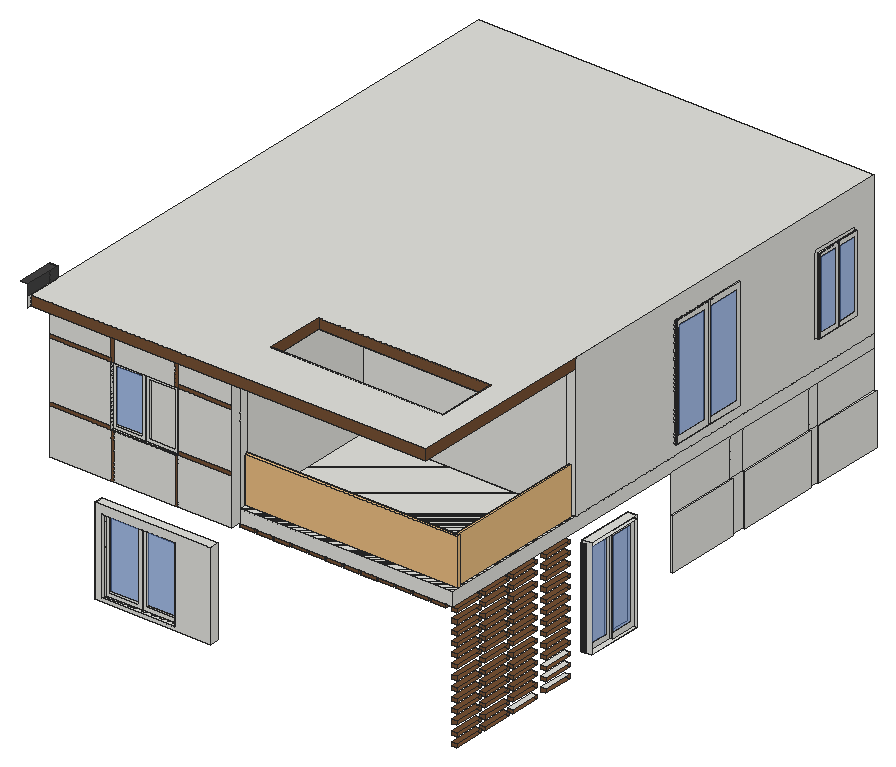
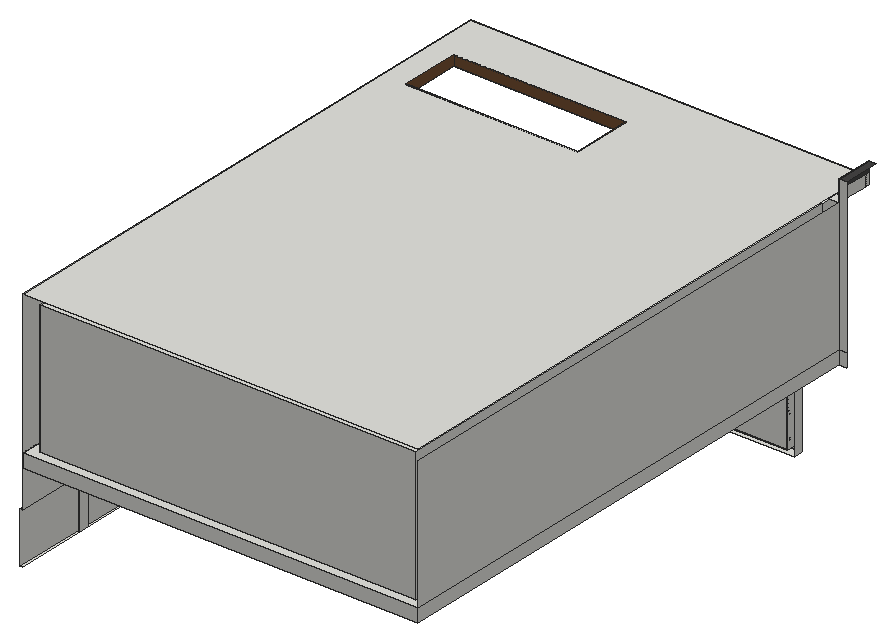
# SketchUp Ruby script. Lengths in inches.
U = 1.inch
M = Sketchup.active_model
def pt(a) = Geom::Point3d.new(a.map { |v| v * U })
def face(e, loops, mat)
  f = e.add_face(loops[0].map { |a| pt(a) })
  loops[1..].each { |l| e.add_face(l.map { |a| pt(a) }).erase! }
  f.material = f.back_material = mat if mat
  f
end
# faces: each face lists its corners as indices into pts; further lists are holes
def faces(e, pts, list, mat = nil) = list.each { |f| face(e, (f[0].is_a?(Array) ? f : [f]).map { |l| l.map { |i| pts[i] } }, mat) }
# xy, xz, yz: faces in a plane at the given z, y or x. An outline is a flat list of corners, or four numbers for a rectangle; further outlines are holes
def ring(l) = l.size == 4 ? [[l[0], l[1]], [l[2], l[1]], [l[2], l[3]], [l[0], l[3]]] : l.each_slice(2).to_a
def flat(e, list, mat, &to3) = list.each { |f| face(e, (f[0].is_a?(Array) ? f : [f]).map { |l| ring(l).map { |u, v| to3.(u, v) } }, mat) }
def xy(e, z, list, mat = nil) = flat(e, list, mat) { |x, y| [x, y, z] }
def xz(e, y, list, mat = nil) = flat(e, list, mat) { |x, z| [x, y, z] }
def yz(e, x, list, mat = nil) = flat(e, list, mat) { |y, z| [x, y, z] }
def lines(e, pts, list) = list.each { |a, b| e.add_line(pt(pts[a]), pt(pts[b])) }
# prism: a flat outline (further loops are holes) pulled along v
def prism(e, loops, v, mat = nil)
  f = face(e, loops, mat); d = Geom::Vector3d.new(v.map { |x| x * U })
  f.pushpull(f.normal.samedirection?(d) ? d.length : -d.length)
end
def box(e, o, s, mat = nil) = prism(e, [[o, [o[0] + s[0], o[1], o[2]], [o[0] + s[0], o[1] + s[1], o[2]], [o[0], o[1] + s[1], o[2]]]], [0, 0, s[2]], mat)
def at(x, y, z, deg = 0) = Geom::Transformation.translation(pt([x, y, z])) * Geom::Transformation.rotation(ORIGIN, Z_AXIS, deg.degrees)
def axes(o, x, y, z) = Geom::Transformation.new([*x, 0, *y, 0, *z, 0, *pt(o).to_a, 1])
def part(name) = M.definitions.add(name)
# library, detail: a bought-in or finely detailed component or shape, given as its bounding box
def library(name, o, s) = part(name).tap { |d| box(d.entities, o, s) }
def detail(e, o, s) = box(e.add_group.entities, o, s)
def put(e, d, t, mat = nil) = e.add_instance(d, t).tap { |i| i.material = mat if mat }
def group(e, t, mat = nil) = e.add_group.tap { |g| g.transformation = t; g.material = mat if mat }.entities
root = M.entities
M.materials.add("[Granite Dark Gray]").color = [69, 68, 68]
M.materials.add("[Sandstone]").color = [118, 81, 52]
M.materials.add("[Translucent Glass Blue]").color = [100, 149, 237]
M.materials["[Translucent Glass Blue]"].alpha = 0.5
c1 = part("Janela aluminio\#1")
xy(c1.entities,0,[[0,0,47.24,1.57],[23.62,1.57,47.24,2.76],[0,2.76,25.98,3.9375],[0,3.9375,47.24,5.91]])
xy(c1.entities,43.31,[[0,0,47.24,1.57],[23.62,1.57,47.24,2.76],[0,2.76,0,5.91,47.24,5.91,47.24,3.9375,25.98,3.9375,25.98,2.76],[25.98,2.76,47.24,3.9375]])
xz(c1.entities,1.57,[[0,0,23.62,0,23.62,41.34,21.26,41.34,21.26,1.97,1.97,1.97,1.97,41.34,23.62,41.34,23.62,43.31,0,43.31],[[23.62,0,47.24,43.31],[25.7,1.97,45.28,41.34]]])
xz(c1.entities,2.76,[[[0,0,23.62,43.31],[2.36,2.36,21.26,40.94]],[23.62,0,25.98,43.31]])
xz(c1.entities,2.76,[[2.36,2.36,21.26,40.94]],"[Translucent Glass Blue]")
xz(c1.entities,3.9375,[[25.98,0,25.98,2.36,44.88,2.36,44.88,40.94,25.98,40.94,25.98,43.31,47.24,43.31,47.24,0]])
xz(c1.entities,3.9375,[[25.98,2.36,44.88,40.94]],"[Translucent Glass Blue]")
yz(c1.entities,0,[[0,0,1.57,43.31],[2.76,0,5.91,43.31]])
yz(c1.entities,23.62,[[1.57,0,2.76,43.31]])
yz(c1.entities,25.98,[[2.76,0,3.9375,43.31]])
yz(c1.entities,47.24,[[0,0,1.57,43.31],[1.57,0,2.76,43.31],[3.9375,0,5.91,43.31]])
c2 = part("Janela aluminio")
xy(c2.entities,0,[[0,0,47.24,1.57],[23.62,1.57,47.24,2.76],[0,2.76,25.98,3.9375],[0,3.9375,47.24,5.91]])
xy(c2.entities,43.31,[[0,0,47.24,1.57],[23.62,1.57,47.24,2.76],[0,2.76,0,5.91,47.24,5.91,47.24,3.9375,25.98,3.9375,25.98,2.76],[25.98,2.76,47.24,3.9375]])
xz(c2.entities,1.57,[[0,0,23.62,0,23.62,41.34,21.26,41.34,21.26,1.97,1.97,1.97,1.97,41.34,23.62,41.34,23.62,43.31,0,43.31],[[23.62,0,47.24,43.31],[25.7,1.97,45.28,41.34]]])
xz(c2.entities,2.76,[[[0,0,23.62,43.31],[2.36,2.36,21.26,40.94]],[23.62,0,25.98,43.31]])
xz(c2.entities,2.76,[[2.36,2.36,21.26,40.94]],"[Translucent Glass Blue]")
xz(c2.entities,3.9375,[[25.98,0,25.98,2.36,44.88,2.36,44.88,40.94,25.98,40.94,25.98,43.31,47.24,43.31,47.24,0]])
xz(c2.entities,3.9375,[[25.98,2.36,44.88,40.94]],"[Translucent Glass Blue]")
yz(c2.entities,0,[[0,0,1.57,43.31],[2.76,0,5.91,43.31]])
yz(c2.entities,23.62,[[1.57,0,2.76,43.31]])
yz(c2.entities,25.98,[[2.76,0,3.9375,43.31]])
yz(c2.entities,47.24,[[0,0,1.57,43.31],[1.57,0,2.76,43.31],[3.9375,0,5.91,43.31]])
c3 = part("Group\#3")
prism(c3.entities,[[[0,0,140.51],[14.1875,0,140.51],[14.1875,0,0],[0,0,0],[0,0,131.51]]],[0,-3,0])
c4 = part("Group\#4")
box(c4.entities,[0,-480,0],[360,480,12])
c5 = library("Wagner Glass Railing",[9.08,102.375,1.53],[2.51,145.5,42.05])
xy(root,24.68,[[374.26,80.89,378.76,108.58],[374.26,112.7,378.76,140.39],[374.26,144.51,378.76,172.2],[374.26,182.01,378.76,209.7]],"[Sandstone]")
xy(root,28.05,[[374.26,144.51,378.76,172.2],[374.26,182.01,378.76,209.7]])
xy(root,28.05,[[374.26,80.89,378.76,108.58],[374.26,112.7,378.76,140.39]],"[Sandstone]")
xy(root,32.94,[[370.32,234.07,378.76,285.88]])
xy(root,33.83,[[374.26,80.89,378.76,108.58],[374.26,112.7,378.76,140.39],[374.26,144.51,378.76,172.2],[374.26,182.01,378.76,209.7]],"[Sandstone]")
xy(root,37.2,[[374.26,182.01,378.76,209.7]])
xy(root,37.2,[[374.26,80.89,378.76,108.58],[374.26,112.7,378.76,140.39],[374.26,144.51,378.76,172.2]],"[Sandstone]")
xy(root,42.98,[[374.26,80.89,378.76,108.58],[374.26,112.7,378.76,140.39],[374.26,144.51,378.76,172.2],[374.26,182.01,378.76,209.7]],"[Sandstone]")
xy(root,46.02,[[66.65,58.66,171.96,67.23]])
xy(root,46.36,[[374.26,182.01,378.76,209.7]])
xy(root,46.36,[[374.26,80.89,378.76,108.58],[374.26,112.7,378.76,140.39],[374.26,144.51,378.76,172.2]],"[Sandstone]")
xy(root,49.26,[[73.08,58.66,139.58,66.23]])
xy(root,52.13,[[374.26,80.89,378.76,108.58],[374.26,112.7,378.76,140.39],[374.26,144.51,378.76,172.2],[374.26,182.01,378.76,209.7]],"[Sandstone]")
xy(root,55.51,[[374.26,80.89,378.76,108.58],[374.26,112.7,378.76,140.39],[374.26,144.51,378.76,172.2],[374.26,182.01,378.76,209.7]],"[Sandstone]")
xy(root,61.25,[[378.76,324.38,380.7,392.06],[378.76,406.38,380.7,481.66],[378.76,490.64,380.7,555.98]])
xy(root,61.29,[[374.26,80.89,378.76,108.58],[374.26,112.7,378.76,140.39],[374.26,144.51,378.76,172.2],[374.26,182.01,378.76,209.7]],"[Sandstone]")
xy(root,64.66,[[374.26,80.89,378.76,108.58],[374.26,112.7,378.76,140.39],[374.26,144.51,378.76,172.2],[374.26,182.01,378.76,209.7]],"[Sandstone]")
xy(root,70.4375,[[374.26,80.89,378.76,108.58],[374.26,112.7,378.76,140.39],[374.26,144.51,378.76,172.2],[374.26,182.01,378.76,209.7]],"[Sandstone]")
xy(root,73.8125,[[374.26,80.89,378.76,108.58],[374.26,112.7,378.76,140.39],[374.26,144.51,378.76,172.2],[374.26,182.01,378.76,209.7]],"[Sandstone]")
xy(root,79.59,[[374.26,80.89,378.76,108.58],[374.26,112.7,378.76,140.39],[374.26,144.51,378.76,172.2],[374.26,182.01,378.76,209.7]],"[Sandstone]")
xy(root,82.97,[[374.26,80.89,378.76,108.58],[374.26,112.7,378.76,140.39],[374.26,144.51,378.76,172.2],[374.26,182.01,378.76,209.7]],"[Sandstone]")
xy(root,88.74,[[374.26,80.89,378.76,108.58],[374.26,112.7,378.76,140.39],[374.26,144.51,378.76,172.2],[374.26,182.01,378.76,209.7]],"[Sandstone]")
xy(root,92.12,[[374.26,80.89,378.76,108.58],[374.26,112.7,378.76,140.39],[374.26,144.51,378.76,172.2],[374.26,182.01,378.76,209.7]],"[Sandstone]")
xy(root,97.9,[[374.26,80.89,378.76,108.58],[374.26,112.7,378.76,140.39],[374.26,144.51,378.76,172.2],[374.26,182.01,378.76,209.7]],"[Sandstone]")
xy(root,101.27,[[374.26,80.89,378.76,108.58],[374.26,112.7,378.76,140.39],[374.26,144.51,378.76,172.2],[374.26,182.01,378.76,209.7]],"[Sandstone]")
xy(root,107.05,[[374.26,80.89,378.76,108.58],[374.26,112.7,378.76,140.39],[374.26,144.51,378.76,172.2],[374.26,182.01,378.76,209.7]],"[Sandstone]")
xy(root,107.78,[[378.76,324.38,380.7,392.06],[378.76,406.38,380.7,481.66],[378.76,490.64,380.7,555.98]])
xy(root,110.42,[[374.26,80.89,378.76,108.58],[374.26,112.7,378.76,140.39],[374.26,144.51,378.76,172.2],[374.26,182.01,378.76,209.7]],"[Sandstone]")
xy(root,116.2,[[374.26,80.89,378.76,108.58],[374.26,112.7,378.76,140.39],[374.26,144.51,378.76,172.2],[374.26,182.01,378.76,209.7]],"[Sandstone]")
xy(root,117.95,[[73.08,58.66,139.58,66.23]])
xy(root,119.58,[[374.26,80.89,378.76,108.58],[374.26,112.7,378.76,140.39],[374.26,144.51,378.76,172.2],[374.26,182.01,378.76,209.7]],"[Sandstone]")
xy(root,124.38,[[370.32,234.07,378.76,285.88]])
xy(root,125.2,[[66.65,58.66,171.96,67.23]])
xy(root,125.35,[[374.26,80.89,378.76,108.58],[374.26,112.7,378.76,140.39],[374.26,144.51,378.76,172.2],[374.26,182.01,378.76,209.7]],"[Sandstone]")
xy(root,128.73,[[374.26,80.89,378.76,108.58],[374.26,112.7,378.76,140.39],[374.26,144.51,378.76,172.2],[374.26,182.01,378.76,209.7]],"[Sandstone]")
xy(root,134.51,[[374.26,80.89,378.76,108.58],[374.26,112.7,378.76,140.39],[374.26,144.51,378.76,172.2],[374.26,182.01,378.76,209.7]],"[Sandstone]")
xy(root,137.88,[[374.26,80.89,378.76,108.58],[374.26,112.7,378.76,140.39],[374.26,144.51,378.76,172.2],[374.26,182.01,378.76,209.7]],"[Sandstone]")
xy(root,141.96,[[[18.76,75.98,184.57,75.98,184.57,216.49,378.76,216.49,378.76,555.98,18.76,555.98],[27.76,84.98,27.76,546.98,369.76,546.98,369.76,225.49,106.14,225.49,106.14,84.98]],[374.26,75.98,378.76,216.49]])
xy(root,153.96,[[[18.76,75.98,18.76,555.98,378.76,555.98,378.76,216.49,184.64,216.49,184.64,84.98,184.57,84.98,184.57,75.98],[27.76,84.98,176.7,84.98,176.7,225.49,369.76,225.49,369.76,546.98,27.76,546.98]],[184.57,75.98,378.76,75.98,378.76,216.49,369.76,216.49,369.76,84.98,184.57,84.98],[184.64,84.98,369.76,216.49]])
xy(root,183.6,[[74.85,67.23,135.04,70.35]])
xy(root,238.54,[[74.85,67.23,135.04,70.35]])
xy(root,273.96,[[18.76,67.23,27.76,75.98],[27.76,67.23,176.7,75.98],[176.7,67.23,184.57,75.98],[27.76,75.98,176.7,84.98],[176.7,75.98,184.57,75.98,184.57,84.98,184.64,84.98,184.64,216.49,369.76,216.49,369.76,225.49,176.7,225.49],
  [27.76,84.98,27.76,546.98,369.76,546.98,369.76,225.49,176.7,225.49,176.7,84.98]])
xy(root,273.96,[[[18.76,45.91,18.76,67.23,184.57,67.23,184.57,84.98,184.64,84.98,184.64,216.49,369.76,216.49,369.76,45.91],[199.77,92.54,356.4,147.73]],[369.76,45.91,378.76,216.49]],"[Sandstone]")
xy(root,283.53,[[[18.76,45.91,378.76,555.98],[199.77,92.54,356.4,147.73]]])
xy(root,293.28,[[11.76,42.54,18.76,75.98]],"[Granite Dark Gray]")
xz(root,45.91,[[18.76,273.96,378.76,283.53]],"[Sandstone]")
xz(root,58.66,[[[66.65,46.02,171.96,125.2],[73.08,49.26,139.58,117.95]]])
xz(root,66.23,[[73.08,49.26,139.58,117.95]])
xz(root,67.23,[[18.76,141.96,74.85,183.6],[77.17,141.96,132.6,183.6],[135.04,141.96,184.57,184.27],[18.76,186.83,74.85,238.54],[135.04,187.49,184.57,238.54],
  [77.17,238.54,132.6,273.96],[18.76,241.77,74.85,273.96],[135.04,241.77,184.57,273.96]])
xz(root,67.23,[[74.85,141.96,77.17,183.6],[132.6,141.96,135.04,183.6],[18.76,183.6,74.85,186.83],[135.04,184.27,184.57,187.49],[18.76,238.54,74.85,241.77],
  [74.85,238.54,77.17,273.96],[132.6,238.54,135.04,273.96],[135.04,238.54,184.57,241.77]],"[Sandstone]")
xz(root,70.35,[[74.85,183.6,135.04,238.54]])
xz(root,75.98,[[11.76,141.96,18.76,153.96],[18.76,141.96,184.57,153.96],[11.76,153.96,18.76,293.28],[18.76,153.96,184.57,273.96]])
xz(root,80.89,[[374.26,24.68,378.76,28.05],[374.26,33.83,378.76,37.2],[374.26,42.98,378.76,46.36],[374.26,52.13,378.76,55.51],[374.26,61.29,378.76,64.66],
  [374.26,70.4375,378.76,73.8125],[374.26,79.59,378.76,82.97],[374.26,88.74,378.76,92.12],[374.26,97.9,378.76,101.27],[374.26,107.05,378.76,110.42],
  [374.26,116.2,378.76,119.58],[374.26,125.35,378.76,128.73],[374.26,134.51,378.76,137.88]],"[Sandstone]")
xz(root,84.98,[[27.76,153.96,176.7,273.96],[184.57,153.96,184.64,273.96]])
xz(root,92.54,[[199.77,273.96,356.4,283.53]],"[Sandstone]")
xz(root,108.58,[[374.26,24.68,378.76,28.05],[374.26,33.83,378.76,37.2],[374.26,42.98,378.76,46.36],[374.26,52.13,378.76,55.51],[374.26,61.29,378.76,64.66],
  [374.26,70.4375,378.76,73.8125],[374.26,79.59,378.76,82.97],[374.26,88.74,378.76,92.12],[374.26,97.9,378.76,101.27],[374.26,107.05,378.76,110.42],
  [374.26,116.2,378.76,119.58],[374.26,125.35,378.76,128.73],[374.26,134.51,378.76,137.88]],"[Sandstone]")
xz(root,112.7,[[374.26,24.68,378.76,28.05],[374.26,33.83,378.76,37.2],[374.26,42.98,378.76,46.36],[374.26,52.13,378.76,55.51],[374.26,61.29,378.76,64.66],
  [374.26,70.4375,378.76,73.8125],[374.26,79.59,378.76,82.97],[374.26,88.74,378.76,92.12],[374.26,97.9,378.76,101.27],[374.26,107.05,378.76,110.42],
  [374.26,116.2,378.76,119.58],[374.26,125.35,378.76,128.73],[374.26,134.51,378.76,137.88]],"[Sandstone]")
xz(root,140.39,[[374.26,24.68,378.76,28.05],[374.26,33.83,378.76,37.2],[374.26,42.98,378.76,46.36],[374.26,52.13,378.76,55.51],[374.26,61.29,378.76,64.66],
  [374.26,70.4375,378.76,73.8125],[374.26,79.59,378.76,82.97],[374.26,88.74,378.76,92.12],[374.26,97.9,378.76,101.27],[374.26,107.05,378.76,110.42],
  [374.26,116.2,378.76,119.58],[374.26,125.35,378.76,128.73],[374.26,134.51,378.76,137.88]],"[Sandstone]")
xz(root,144.51,[[374.26,24.68,378.76,28.05],[374.26,33.83,378.76,37.2],[374.26,42.98,378.76,46.36],[374.26,52.13,378.76,55.51],[374.26,61.29,378.76,64.66],
  [374.26,70.4375,378.76,73.8125],[374.26,79.59,378.76,82.97],[374.26,88.74,378.76,92.12],[374.26,97.9,378.76,101.27],[374.26,107.05,378.76,110.42],
  [374.26,116.2,378.76,119.58],[374.26,125.35,378.76,128.73],[374.26,134.51,378.76,137.88]],"[Sandstone]")
xz(root,147.73,[[199.77,273.96,356.4,283.53]],"[Sandstone]")
xz(root,172.2,[[374.26,24.68,378.76,28.05],[374.26,33.83,378.76,37.2],[374.26,42.98,378.76,46.36],[374.26,52.13,378.76,55.51],[374.26,61.29,378.76,64.66],
  [374.26,70.4375,378.76,73.8125],[374.26,79.59,378.76,82.97],[374.26,88.74,378.76,92.12],[374.26,97.9,378.76,101.27],[374.26,107.05,378.76,110.42],
  [374.26,116.2,378.76,119.58],[374.26,125.35,378.76,128.73],[374.26,134.51,378.76,137.88]],"[Sandstone]")
xz(root,182.01,[[374.26,24.68,378.76,28.05],[374.26,33.83,378.76,37.2],[374.26,42.98,378.76,46.36],[374.26,52.13,378.76,55.51],[374.26,61.29,378.76,64.66],
  [374.26,70.4375,378.76,73.8125],[374.26,79.59,378.76,82.97],[374.26,88.74,378.76,92.12],[374.26,97.9,378.76,101.27],[374.26,107.05,378.76,110.42],
  [374.26,116.2,378.76,119.58],[374.26,125.35,378.76,128.73],[374.26,134.51,378.76,137.88]],"[Sandstone]")
xz(root,209.7,[[374.26,24.68,378.76,28.05],[374.26,33.83,378.76,37.2],[374.26,42.98,378.76,46.36],[374.26,52.13,378.76,55.51],[374.26,61.29,378.76,64.66],
  [374.26,70.4375,378.76,73.8125],[374.26,79.59,378.76,82.97],[374.26,88.74,378.76,92.12],[374.26,97.9,378.76,101.27],[374.26,107.05,378.76,110.42],
  [374.26,116.2,378.76,119.58],[374.26,125.35,378.76,128.73],[374.26,134.51,378.76,137.88]],"[Sandstone]")
xz(root,216.49,[[184.64,153.96,369.76,273.96],[369.76,153.96,378.76,273.96]])
xz(root,225.49,[[176.7,153.96,369.76,273.96]])
xz(root,234.07,[[370.32,32.94,378.76,124.38]])
xz(root,285.88,[[370.32,32.94,378.76,124.38]])
xz(root,324.38,[[378.76,61.25,380.7,107.78]])
xz(root,392.06,[[378.76,61.25,380.7,107.78]])
xz(root,406.38,[[378.76,61.25,380.7,107.78]])
xz(root,481.66,[[378.76,61.25,380.7,107.78]])
xz(root,490.64,[[378.76,61.25,380.7,107.78]])
xz(root,546.98,[[27.76,153.96,369.76,273.96]])
yz(root,18.76,[[75.98,153.96,555.98,273.96],[42.54,273.96,45.91,283.53],[45.91,273.96,67.23,283.53],[67.23,273.96,75.98,283.53]])
yz(root,18.76,[[42.54,283.53,67.23,293.28],[67.23,283.53,75.98,293.28]],"[Granite Dark Gray]")
yz(root,27.76,[[84.98,153.96,546.98,273.96]])
yz(root,66.65,[[58.66,46.02,67.23,125.2]])
yz(root,73.08,[[58.66,49.26,66.23,117.95]])
yz(root,74.85,[[67.23,183.6,70.35,238.54]])
yz(root,135.04,[[67.23,183.6,70.35,238.54]])
yz(root,139.58,[[58.66,49.26,66.23,117.95]])
yz(root,171.96,[[58.66,46.02,67.23,125.2]])
yz(root,176.7,[[84.98,153.96,225.49,273.96]])
yz(root,184.57,[[67.23,141.96,75.98,273.96],[75.98,153.96,84.98,273.96]])
yz(root,184.64,[[84.98,153.96,216.49,273.96]])
yz(root,199.77,[[92.54,273.96,147.73,283.53]],"[Sandstone]")
yz(root,356.4,[[92.54,273.96,147.73,283.53]],"[Sandstone]")
yz(root,369.76,[[225.49,153.96,546.98,273.96]])
yz(root,370.32,[[234.07,32.94,285.88,124.38]])
yz(root,378.76,[[392.06,61.25,406.38,107.78],[481.66,61.25,490.64,107.78],[324.38,107.78,392.06,141.96],[392.06,107.78,406.38,141.96],[406.38,107.78,481.66,141.96],
  [481.66,107.78,490.64,141.96],[490.64,107.78,555.98,141.96],[[216.49,153.96,555.98,283.53],[327.52,163.4,401.46,264.78],[488.76,179.61,532.82,250.9]],[327.52,163.4,401.46,264.78],[488.76,179.61,532.82,250.9]])
yz(root,378.76,[[45.91,273.96,216.49,283.53]],"[Sandstone]")
yz(root,380.7,[[324.38,61.25,392.06,107.78],[406.38,61.25,481.66,107.78],[490.64,61.25,555.98,107.78]])
put(root,c1,axes([369.45,234.07,121.71],[0,1.0967,0],[1.5769,0,0],[0,0,-2.04982]))
put(root,c2,axes([73.08,61.72,49.26],[1.40758,0,0],[0,1,0],[0,0,1.5777]))
put(root,c3,axes([184.57,216.49,141.96],[1,0,0],[0,0,1],[0,-1,0]),"[Sandstone]")
put(root,c3,axes([200.39,216.49,141.96],[1,0,0],[0,0,1],[0,-1,0]),"[Sandstone]")
put(root,c3,axes([216.2,216.49,141.96],[1,0,0],[0,0,1],[0,-1,0]),"[Sandstone]")
put(root,c3,axes([232.01,216.49,141.96],[1,0,0],[0,0,1],[0,-1,0]),"[Sandstone]")
put(root,c3,axes([247.82,216.49,141.96],[1,0,0],[0,0,1],[0,-1,0]),"[Sandstone]")
put(root,c3,axes([263.64,216.49,141.96],[1,0,0],[0,0,1],[0,-1,0]),"[Sandstone]")
put(root,c3,axes([279.45,216.49,141.96],[1,0,0],[0,0,1],[0,-1,0]),"[Sandstone]")
put(root,c3,axes([295.26,216.49,141.96],[1,0,0],[0,0,1],[0,-1,0]),"[Sandstone]")
put(root,c3,axes([311.07,216.49,141.96],[1,0,0],[0,0,1],[0,-1,0]),"[Sandstone]")
put(root,c3,axes([326.89,216.49,141.96],[1,0,0],[0,0,1],[0,-1,0]),"[Sandstone]")
put(root,c3,axes([342.7,216.49,141.96],[1,0,0],[0,0,1],[0,-1,0]),"[Sandstone]")
put(root,c3,axes([358.51,216.49,141.96],[1,0,0],[0,0,1],[0,-1,0]),"[Sandstone]")
put(root,c4,at(18.76,555.98,141.96))
put(root,c5,axes([514.13,73.38,152.43],[0,1,0],[-1.32953,0,0],[0,0,1]))
put(root,c5,axes([364.63,-6.68,152.43],[1,0,0],[0,0.89153,0],[0,0,1]))
put(root,c1,axes([379.01,328.84,264.78],[0,1.53711,0],[0.22222,0,0],[0,0,-2.34084]))
put(root,c1,axes([380.45,489.87,249.16],[0,0.90911,0],[0.22222,0,0],[0,0,-1.60599]))
put(root,c2,axes([74.85,67.23,184.27],[1.27397,0,0],[0,1,0],[0,0,1.25324]))
